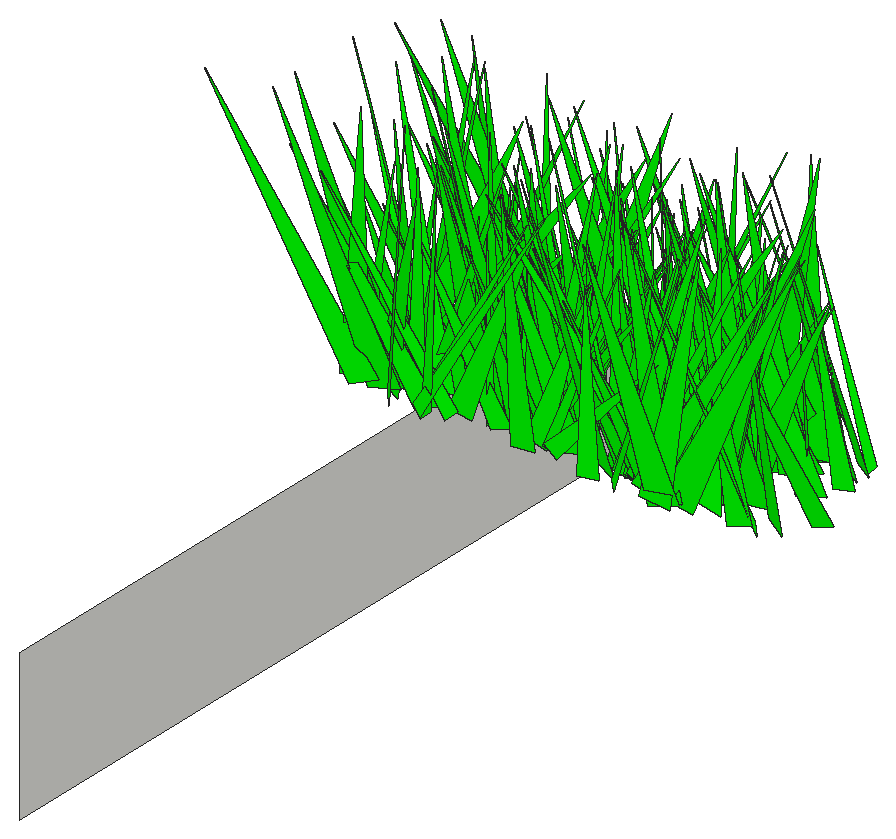
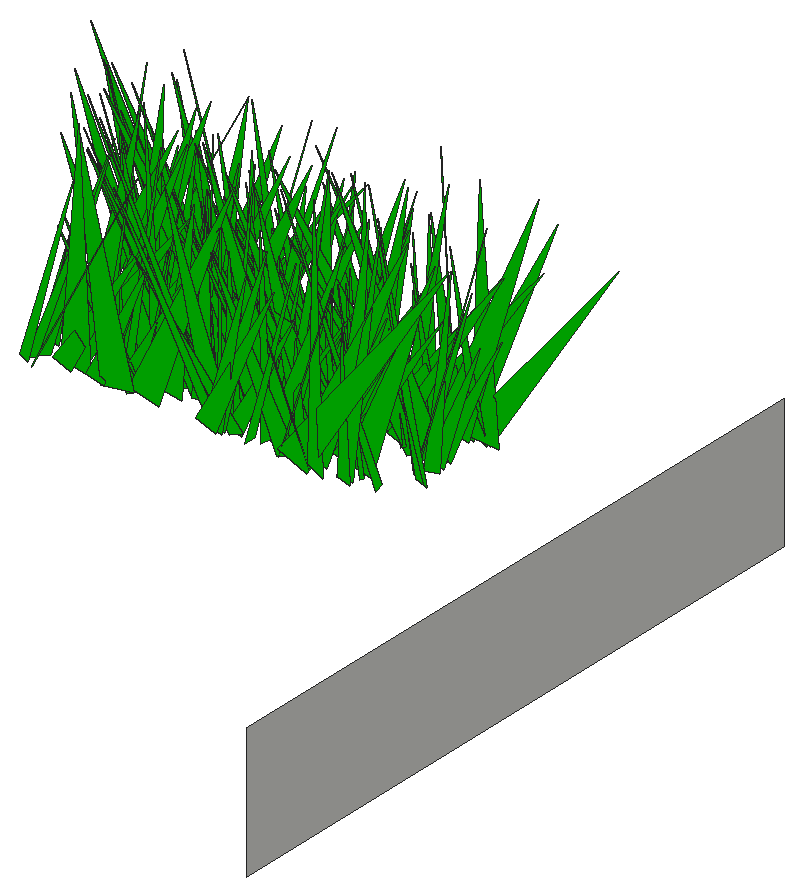
# SketchUp Ruby script. Lengths in inches.
U = 1.inch
M = Sketchup.active_model
def pt(a) = Geom::Point3d.new(a.map { |v| v * U })
def face(e, loops, mat)
  f = e.add_face(loops[0].map { |a| pt(a) })
  loops[1..].each { |l| e.add_face(l.map { |a| pt(a) }).erase! }
  f.material = f.back_material = mat if mat
  f
end
# faces: each face lists its corners as indices into pts; further lists are holes
def faces(e, pts, list, mat = nil) = list.each { |f| face(e, (f[0].is_a?(Array) ? f : [f]).map { |l| l.map { |i| pts[i] } }, mat) }
# xy, xz, yz: faces in a plane at the given z, y or x. An outline is a flat list of corners, or four numbers for a rectangle; further outlines are holes
def ring(l) = l.size == 4 ? [[l[0], l[1]], [l[2], l[1]], [l[2], l[3]], [l[0], l[3]]] : l.each_slice(2).to_a
def flat(e, list, mat, &to3) = list.each { |f| face(e, (f[0].is_a?(Array) ? f : [f]).map { |l| ring(l).map { |u, v| to3.(u, v) } }, mat) }
def xy(e, z, list, mat = nil) = flat(e, list, mat) { |x, y| [x, y, z] }
def xz(e, y, list, mat = nil) = flat(e, list, mat) { |x, z| [x, y, z] }
def yz(e, x, list, mat = nil) = flat(e, list, mat) { |y, z| [x, y, z] }
def lines(e, pts, list) = list.each { |a, b| e.add_line(pt(pts[a]), pt(pts[b])) }
# prism: a flat outline (further loops are holes) pulled along v
def prism(e, loops, v, mat = nil)
  f = face(e, loops, mat); d = Geom::Vector3d.new(v.map { |x| x * U })
  f.pushpull(f.normal.samedirection?(d) ? d.length : -d.length)
end
def box(e, o, s, mat = nil) = prism(e, [[o, [o[0] + s[0], o[1], o[2]], [o[0] + s[0], o[1] + s[1], o[2]], [o[0], o[1] + s[1], o[2]]]], [0, 0, s[2]], mat)
def at(x, y, z, deg = 0) = Geom::Transformation.translation(pt([x, y, z])) * Geom::Transformation.rotation(ORIGIN, Z_AXIS, deg.degrees)
def axes(o, x, y, z) = Geom::Transformation.new([*x, 0, *y, 0, *z, 0, *pt(o).to_a, 1])
def part(name) = M.definitions.add(name)
# library, detail: a bought-in or finely detailed component or shape, given as its bounding box
def library(name, o, s) = part(name).tap { |d| box(d.entities, o, s) }
def detail(e, o, s) = box(e.add_group.entities, o, s)
def put(e, d, t, mat = nil) = e.add_instance(d, t).tap { |i| i.material = mat if mat }
def group(e, t, mat = nil) = e.add_group.tap { |g| g.transformation = t; g.material = mat if mat }.entities
root = M.entities
M.materials.add("[0065_Lime]").color = [0, 255, 0]
c1 = part("fur_instance\#9")
p = [[0.8125,0,1.79],[0.67,-0.02,1.48],[0,-0.11,0],[0,0.11,0]]
faces(c1.entities,p,[[0,1,2,3]])
yz(root,5.71,[[0,-11.8125,39.75,-3.9375]])
put(root,c1,axes([8.52,19.14,1.48],[-4.51597,1.0152,0.75582],[-6.76232,-0.52719,-3.00512],[-2.70756,-0.37656,6.24484]),"[0065_Lime]")
put(root,c1,axes([9.53,19.26,1.48],[-0.92745,-1.18344,1.15572],[8.13091,-0.06085,2.2291],[-2.61483,0.23052,6.52155]),"[0065_Lime]")
put(root,c1,axes([8.54,21.75,1.48],[0.14236,-0.67611,0.80396],[4.52504,0.07211,1.50186],[-1.91106,0.12037,3.61603]),"[0065_Lime]")
put(root,c1,axes([8.66,23.4,1.48],[-8.88567,-0.25424,1.35395],[1.25522,-1.22333,-2.24699],[2.11392,-0.34227,7.02545]),"[0065_Lime]")
put(root,c1,axes([8.39,22.4,1.48],[-0.17151,-0.64742,0.31901],[4.46442,-0.00882,0.98829],[-1.20447,0.0595,3.61774]),"[0065_Lime]")
put(root,c1,axes([9.04,22.44,1.48],[-6.57212,0.41088,0.28365],[-2.7373,-0.89658,1.55629],[1.0858,0.22672,5.64032]),"[0065_Lime]")
put(root,c1,axes([9.7,19.55,1.48],[-0.1146,-1.28054,1.0583],[8.86048,0.03424,2.02291],[-2.49622,0.18031,7.13186]),"[0065_Lime]")
put(root,c1,axes([8.04,23.1,1.48],[-4.80678,-0.70041,0.91441],[4.7596,-0.69264,-1.22373],[1.85882,-0.03767,5.49804]),"[0065_Lime]")
put(root,c1,axes([11.95,19.03,1.48],[-4.72071,0.76903,0.39332],[-5.14246,-0.58693,-2.38257],[-1.93422,-0.31647,5.37455]),"[0065_Lime]")
put(root,c1,axes([7.86,19.42,1.48],[5.30316,-0.969,1.02],[6.74982,0.76558,1.15187],[-1.88838,0.01526,6.98171]),"[0065_Lime]")
put(root,c1,axes([10.86,25.02,1.48],[-2.71894,-1.0235,1.49211],[7.41679,-0.32251,1.5292],[-1.18715,0.32924,6.13636]),"[0065_Lime]")
put(root,c1,axes([8.25,19.28,1.48],[5.38611,0.66899,0.37338],[-4.41146,0.73237,-1.86579],[-1.84817,0.2015,5.54166]),"[0065_Lime]")
put(root,c1,axes([12.25,21.2,1.48],[-0.93493,-0.96245,1.99029],[6.42475,0.0532,2.8589],[-3.40916,0.3642,4.84194]),"[0065_Lime]")
put(root,c1,axes([7.98,24.05,1.48],[7.33829,0.65143,1.33023],[-4.37612,1.05375,-1.31921],[-2.23967,0.07548,6.9361]),"[0065_Lime]")
put(root,c1,axes([12.09,24.75,1.48],[-4.89413,0.62544,0.37384],[-4.32649,-0.637,-1.76465],[-1.14195,-0.26712,5.0835]),"[0065_Lime]")
put(root,c1,axes([13.77,26.3,1.48],[-3.51472,-1.22749,0.2766],[8.07714,-0.43627,3.03249],[-3.34436,0.23638,7.03326]),"[0065_Lime]")
put(root,c1,axes([11.29,21.7,1.48],[-1.10307,-0.63213,1.01067],[4.39567,-0.08044,1.48842],[-1.56819,0.21918,3.46114]),"[0065_Lime]")
put(root,c1,axes([7.87,24.19,1.48],[9.02923,-0.23707,1.46941],[1.26598,1.26925,1.71479],[-2.12296,-0.25139,7.27216]),"[0065_Lime]")
put(root,c1,axes([10.75,26.15,1.48],[-6.90175,-0.73018,1.53288],[5.0802,-1.00487,-0.90557],[2.17833,0.03003,6.96867]),"[0065_Lime]")
put(root,c1,axes([13.17,19.14,1.48],[-6.55039,0.35414,0.43805],[-2.49164,-0.81745,-2.50688],[-0.65837,-0.42978,5.12908]),"[0065_Lime]")
put(root,c1,axes([9.55,20.76,1.48],[5.24517,0.61285,0.37116],[-3.95773,0.70463,-1.98125],[-1.8885,0.22546,5.18298]),"[0065_Lime]")
put(root,c1,axes([11.61,20.6,1.48],[-8.02681,0.63334,1.21574],[-4.33342,-1.14566,1.0688],[1.94162,0.06133,7.41134]),"[0065_Lime]")
put(root,c1,axes([12,23.47,1.48],[0.00491,-0.81088,1.79265],[5.85718,0.09899,1.48978],[-1.96232,0.29344,4.45122]),"[0065_Lime]")
put(root,c1,axes([13.33,25.51,1.48],[-2.13529,1.23511,1.47302],[-8.6321,-0.21112,-2.34727],[-2.45463,-0.33197,6.97314]),"[0065_Lime]")
put(root,c1,axes([13.64,24.76,1.48],[-2.97825,-0.76492,0.9224],[5.21144,-0.32095,2.21457],[-1.93893,0.31228,4.53548]),"[0065_Lime]")
put(root,c1,axes([9.54,19.4,1.48],[-4.12303,-0.93043,0.23604],[5.76195,-0.52692,-3.00694],[3.2753,-0.24428,5.58699]),"[0065_Lime]")
put(root,c1,axes([10.28,20.8125,1.48],[-1.74906,-0.67558,0.04949],[4.57049,-0.23643,-1.27519],[1.49314,-0.06767,3.96131]),"[0065_Lime]")
put(root,c1,axes([10.2,18.69,1.48],[-7.80887,-0.33604,3.12821],[1.23428,-1.19432,-2.26054],[4.35726,-0.26392,6.24658]),"[0065_Lime]")
put(root,c1,axes([10.73,19.87,1.48],[-5.16109,0.39853,3.17519],[-4.06968,-0.79103,-1.04984],[2.59212,-0.44843,4.67376]),"[0065_Lime]")
put(root,c1,axes([10.71,26.29,1.48],[4.13664,-0.44364,0.53641],[2.83698,0.57217,1.38184],[-1.53443,-0.13814,4.00095]),"[0065_Lime]")
put(root,c1,axes([10.16,25.64,1.48],[5.76638,0.14354,1.65664],[-1.58452,0.81226,1.29083],[-1.6373,-0.28053,4.58525]),"[0065_Lime]")
put(root,c1,axes([12.85,22.17,1.48],[2.25168,1.20305,2.13517],[-8.5324,0.40368,-1.66827],[-2.71834,-0.27056,7.00502]),"[0065_Lime]")
put(root,c1,axes([10.55,22.08,1.48],[3.82403,0.16991,1.08744],[-1.59634,0.52385,0.97141],[-0.83732,-0.22273,3.11433]),"[0065_Lime]")
put(root,c1,axes([12.38,24.16,1.48],[3.26238,1.02924,2.0799],[-7.34786,0.535,-1.24568],[-2.48954,-0.23028,6.40217]),"[0065_Lime]")
put(root,c1,axes([8.72,22.16,1.48],[2.49265,1.12942,1.40234],[-7.98484,0.27249,2.03678],[1.95376,-0.32729,6.535]),"[0065_Lime]")
put(root,c1,axes([11.73,22.16,1.48],[-5.38252,-0.24176,1.5364],[0.68863,-0.73331,-2.27042],[2.46041,-0.32365,3.99656]),"[0065_Lime]")
put(root,c1,axes([11.08,24.76,1.48],[5.87705,-0.3291,0.76024],[1.70229,0.76351,2.36835],[-1.86039,-0.34103,4.56871]),"[0065_Lime]")
put(root,c1,axes([12.29,18.54,1.48],[5.85026,0.55929,0.97233],[-3.04973,0.77481,-2.7932],[-2.8231,0.32199,5.03236]),"[0065_Lime]")
put(root,c1,axes([12.02,21.33,1.48],[3.45962,0.59945,0.27658],[-4.04081,0.4778,-1.25847],[-1.40947,0.10159,4.28681]),"[0065_Lime]")
put(root,c1,axes([9.04,25.82,1.48],[9.00581,0.29151,1.30551],[-2.57623,1.13462,3.2688],[-0.49281,-0.6041,6.7694]),"[0065_Lime]")
put(root,c1,axes([13.5625,23.2,1.48],[0.41564,-0.69447,0.03329],[4.68844,0.05723,1.27394],[-1.56396,-0.01301,3.82785]),"[0065_Lime]")
put(root,c1,axes([14.9,20.67,1.48],[-9.0282,-0.11103,1.59013],[1.50199,-1.18634,2.8667],[1.47982,0.52675,6.79149]),"[0065_Lime]")
put(root,c1,axes([13.49,20.99,1.48],[2.41747,-1.08088,0.01398],[7.39832,0.32741,1.79122],[-2.10575,-0.09056,6.30927]),"[0065_Lime]")
put(root,c1,axes([9.15,21.7,1.48],[2.60344,0.683,0.40678],[-4.0014,0.25231,2.74862],[2.80439,-0.27406,3.5442]),"[0065_Lime]")
put(root,c1,axes([12.3,26.41,1.48],[8.37035,-0.55491,1.57527],[2.96399,1.14389,3.08182],[-3.24961,-0.38598,6.86854]),"[0065_Lime]")
put(root,c1,axes([14.71,25.96,1.48],[-6.89277,0.09509,0.79888],[-0.3282,-0.92938,1.83337],[1.14666,0.3056,5.32696]),"[0065_Lime]")
put(root,c1,axes([13.4,23.63,1.48],[-4.04851,-0.00151,1.22127],[0.64281,-0.55006,1.38709],[1.3569,0.25608,2.98674]),"[0065_Lime]")
put(root,c1,axes([15.44,19.57,1.48],[-2.28354,0.71758,0.28524],[-4.82771,-0.28399,-1.63183],[-1.70136,-0.15729,4.24757]),"[0065_Lime]")
put(root,c1,axes([10.88,20.86,1.48],[7.55042,-0.47397,0.27797],[3.24255,1.04379,1.36389],[-0.99004,-0.19613,6.58688]),"[0065_Lime]")
put(root,c1,axes([16.12,20.47,1.48],[-3.81413,-0.77301,1.85642],[5.88572,-0.43097,1.98756],[-0.91089,0.45206,5.06931]),"[0065_Lime]")
put(root,c1,axes([13.43,22.12,1.48],[4.49135,-0.41416,0.66232],[2.59175,0.6235,1.436],[-1.62259,-0.15048,4.12702]),"[0065_Lime]")
put(root,c1,axes([13.64,23.21,1.48],[-4.1807,0.3084,1.23402],[-1.6634,-0.61111,1.389],[2.086,0.13077,3.58078]),"[0065_Lime]")
put(root,c1,axes([10.24,21.75,1.48],[4.09063,0.70798,0.20575],[-4.5194,0.49397,2.49387],[2.2415,-0.29608,4.65274]),"[0065_Lime]")
put(root,c1,axes([9.5625,22.0625,1.48],[2.5963,1.09286,2.35775],[-7.43893,0.11711,3.60096],[3.68129,-0.53412,5.61375]),"[0065_Lime]")
put(root,c1,axes([12.93,26.23,1.48],[4.17456,0.20644,0.24318],[-1.28002,0.55547,-1.26266],[-0.78058,0.19317,3.37107]),"[0065_Lime]")
put(root,c1,axes([14.375,20.41,1.48],[6.01675,0.77907,1.63573],[-4.94463,0.88638,-2.1125],[-3.21463,0.09478,6.31094]),"[0065_Lime]")
put(root,c1,axes([13.99,23.44,1.48],[4.68309,0.12287,2.12125],[-1.719,0.6956,1.16081],[-2.1472,-0.2889,3.69717]),"[0065_Lime]")
put(root,c1,axes([15.82,24.58,1.48],[-2.8334,-0.89119,1.44388],[6.54685,-0.3516,1.22824],[-0.71622,0.31162,5.51512]),"[0065_Lime]")
put(root,c1,axes([16.13,20.16,1.48],[-4.02935,-0.9593,2.013],[7.24625,-0.50535,1.52712],[-0.47165,0.43143,6.26472]),"[0065_Lime]")
put(root,c1,axes([16.54,24.29,1.48],[-5.49409,0.14275,0.08975],[-1.00323,-0.7374,-1.3325],[-0.19417,-0.22909,4.34498]),"[0065_Lime]")
put(root,c1,axes([11.63,18.93,1.48],[6.96665,0.31379,0.36258],[-2.27528,0.95111,1.3437],[0.09165,-0.24008,5.79707]),"[0065_Lime]")
put(root,c1,axes([14.69,19.83,1.48],[5.57745,-0.27415,1.43426],[1.19173,0.78139,1.93868],[-2.34423,-0.25504,4.39799]),"[0065_Lime]")
put(root,c1,axes([16.5,26.02,1.48],[-7.04698,0.30872,0.64956],[-1.89783,-0.96364,1.72416],[1.36483,0.25402,5.75134]),"[0065_Lime]")
put(root,c1,axes([14.49,24.81,1.48],[-2.29166,-0.51115,0.22563],[3.31371,-0.3109,-1.3328],[1.52593,-0.09249,3.23316]),"[0065_Lime]")
put(root,c1,axes([17.05,20.16,1.48],[-3.17395,-0.57364,0.51178],[4.07145,-0.4157,1.09338],[-0.6961,0.18419,4.06157]),"[0065_Lime]")
put(root,c1,axes([11.74,18.625,1.48],[7.66634,0.35493,0.19048],[-2.50408,1.04211,1.61392],[0.40557,-0.2749,6.3642]),"[0065_Lime]")
put(root,c1,axes([13.32,19.49,1.48],[4.55521,-0.7039,0.8959],[5.12184,0.61336,-1.08206],[0.27057,0.23968,5.40009]),"[0065_Lime]")
put(root,c1,axes([16.33,23.36,1.48],[7.70292,-0.44018,2.74672],[1.5377,1.11728,3.14665],[-4.3418,-0.38524,5.98747]),"[0065_Lime]")
put(root,c1,axes([12.02,23.78,1.48],[5.7024,0.51738,0.07898],[-3.36031,0.72049,2.37175],[1.50814,-0.35092,4.98591]),"[0065_Lime]")
put(root,c1,axes([15.87,25.56,1.48],[6.42184,-0.14988,2.81865],[2.12568,0.95797,-1.49745],[-2.93715,0.36562,5.07901]),"[0065_Lime]")
put(root,c1,axes([14.69,23.95,1.48],[-0.98557,1.08875,0.87105],[-7.6069,-0.16872,1.372],[1.82083,-0.11556,6.2033]),"[0065_Lime]")
put(root,c1,axes([16.68,24.31,1.48],[-5.48029,-0.51583,0.37851],[3.28972,-0.73269,-1.9446],[1.6941,-0.24588,5.0006]),"[0065_Lime]")
put(root,c1,axes([17.65,25.78,1.48],[-1.66406,-0.64022,0.09718],[4.42274,-0.22251,0.98748],[-1.10098,0.07381,3.81991]),"[0065_Lime]")
put(root,c1,axes([16,21.53,1.48],[3.40175,-1.04621,0.40794],[7.31725,0.48285,1.12339],[-1.46396,-0.01762,6.5629]),"[0065_Lime]")
put(root,c1,axes([12.69,24.53,1.48],[4.62258,-1.01151,0.2415],[7.00165,0.61904,-1.79019],[1.69797,0.20113,6.72445]),"[0065_Lime]")
put(root,c1,axes([13.9,21.72,1.48],[3.47793,-0.48907,0.50837],[3.40501,0.42994,-1.55281],[0.95405,0.24839,3.68875]),"[0065_Lime]")
put(root,c1,axes([17.74,20.77,1.48],[-6.59474,-0.29254,0.84748],[1.81984,-0.92208,-1.29581],[1.45182,-0.17299,5.47391]),"[0065_Lime]")
put(root,c1,axes([17.17,18.83,1.48],[3.20094,0.84632,2.02875],[-6.13144,0.52346,-0.91648],[-2.21378,-0.22611,5.47176]),"[0065_Lime]")
put(root,c1,axes([14.18,26.12,1.48],[3.04422,-0.76222,0.33004],[5.28546,0.39905,-1.37437],[1.28548,0.16429,4.86937]),"[0065_Lime]")
put(root,c1,axes([19.07,19.81,1.48],[-2.15391,0.85559,1.06284],[-6.02122,-0.23654,-1.69296],[-1.58939,-0.26337,4.97324]),"[0065_Lime]")
put(root,c1,axes([18.95,26.2,1.48],[-0.24233,0.79074,1.33555],[-5.42007,0.05773,-1.79607],[-2.23285,-0.22596,4.21486]),"[0065_Lime]")
put(root,c1,axes([18.57,20.2,1.48],[2.6144,0.97004,2.07295],[-6.70575,0.47056,-1.78289],[-3.03038,-0.20439,5.73364]),"[0065_Lime]")
put(root,c1,axes([14.93,23.24,1.48],[0.60212,0.75738,0.49855],[-5.05075,0.04666,1.6609],[1.97915,-0.11135,4.08692]),"[0065_Lime]")
put(root,c1,axes([18.52,26.09,1.48],[-4.33642,0.6658,1.51044],[-5.0832,-0.58317,-1.04194],[0.24485,-0.31512,5.11962]),"[0065_Lime]")
put(root,c1,axes([18.59,26.18,1.48],[0.96901,0.76025,1.42682],[-5.43354,0.19764,-1.0872],[-1.68099,-0.20058,4.3367]),"[0065_Lime]")
put(root,c1,axes([16.92,23.49,1.48],[5.89619,0.791,0.90812],[-5.37717,0.84006,-1.41937],[-2.005,0.07319,6.47712]),"[0065_Lime]")
put(root,c1,axes([15.11,25.13,1.48],[5.44388,-0.9912,1.83413],[7.39986,0.71269,-1.62604],[0.28992,0.42147,7.063]),"[0065_Lime]")
put(root,c1,axes([18.28,22.1,1.48],[1.21948,-1.0478,0.48649],[7.36376,0.18314,1.00402],[-1.3172,0.05374,6.06339]),"[0065_Lime]")
put(root,c1,axes([13.87,24.05,1.48],[8.12448,0.55349,0.5173],[-3.95019,1.08727,2.06616],[0.56173,-0.35938,7.04766]),"[0065_Lime]")
put(root,c1,axes([18.51,22.11,1.48],[4.9532,0.68925,0.32577],[-3.78832,0.58496,-3.36104],[-3.14147,0.38135,4.56675]),"[0065_Lime]")
put(root,c1,axes([21.12,20.95,1.48],[-7.61214,0.41528,0.77912],[-3.10394,-1.00153,-2.17679],[-0.1316,-0.39898,6.27527]),"[0065_Lime]")
put(root,c1,axes([16.91,20.72,1.48],[6.07858,0.79409,0.71559],[-5.49002,0.86072,-1.15017],[-1.60306,0.06339,6.6524]),"[0065_Lime]")
put(root,c1,axes([18.42,25.09,1.48],[8.11333,-0.28978,2.87345],[0.54432,1.16931,2.93449],[-4.05407,-0.42292,6.14458]),"[0065_Lime]")
put(root,c1,axes([21.22,22.83,1.48],[-0.0959,1.26545,2.06522],[-8.71312,0.11796,-2.6897],[-3.41024,-0.33697,6.81409]),"[0065_Lime]")
put(root,c1,axes([18.42,24.93,1.48],[-4.0699,0.59218,1.00747],[-4.03607,-0.59779,0.98637],[1.73333,-0.00149,4.66234]),"[0065_Lime]")
put(root,c1,axes([17.75,20.57,1.48],[-2.38096,0.7267,0.44801],[-4.87591,-0.34152,1.41733],[1.80943,0.03594,4.40882]),"[0065_Lime]")
put(root,c1,axes([15.7,24.66,1.48],[5.71354,0.41429,0.15378],[-2.91512,0.78116,1.14195],[0.48012,-0.18727,5.10356]),"[0065_Lime]")
put(root,c1,axes([17.34,19.51,1.48],[0.09973,0.74013,1.16518],[-5.26071,-0.04067,1.16348],[1.45594,-0.19763,4.12416]),"[0065_Lime]")
put(root,c1,axes([16.4,23.3,1.48],[3.50553,0.60675,0.37787],[-4.21361,0.45487,1.38897],[1.05165,-0.19999,4.30553]),"[0065_Lime]")
put(root,c1,axes([17.16,20.46,1.48],[2.50517,-0.48253,0.39816],[3.38299,0.32114,-1.04162],[0.76627,0.15974,3.2969]),"[0065_Lime]")
put(root,c1,axes([20.96,19.52,1.48],[-7.43308,-0.74265,0.09237],[5.10424,-1.01544,-1.80452],[1.37541,-0.24511,7.19589]),"[0065_Lime]")
put(root,c1,axes([17.08,21.82,1.48],[4.51394,-0.4487,0.47947],[3.2111,0.59576,-1.31974],[0.48227,0.23291,4.29952]),"[0065_Lime]")
put(root,c1,axes([23.86,19.72,1.48],[-7.55702,0.55256,0.45368],[-3.66216,-0.90423,-3.45697],[-1.53717,-0.56225,6.00549]),"[0065_Lime]")
put(root,c1,axes([19.38,22.55,1.48],[5.89257,-0.70031,1.82599],[4.81059,0.88466,1.09782],[-2.59528,0.04976,6.18081]),"[0065_Lime]")
put(root,c1,axes([22.67,22.89,1.48],[-6.39879,0.95966,0.60157],[-6.83825,-0.87635,-1.28002],[-0.65348,-0.22642,7.50414]),"[0065_Lime]")
put(root,c1,axes([21.78,19.8125,1.48],[-9.09715,0.09459,1.29901],[-0.39391,-1.28059,1.29956],[1.68771,0.21099,7.30528]),"[0065_Lime]")
put(root,c1,axes([22.33,19.67,1.48],[-4.416,-0.64604,0.07079],[4.48389,-0.6012,1.21621],[-1.01984,0.15413,5.04075]),"[0065_Lime]")
put(root,c1,axes([17.12,21.49,1.48],[6.70773,0.00986,0.12097],[-0.02769,0.90829,-1.46372],[-0.16207,0.2527,5.25646]),"[0065_Lime]")
put(root,c1,axes([22.09,19.85,1.48],[-1.79777,-0.88309,0.27518],[6.01526,-0.22655,1.63889],[-1.85121,0.12145,5.05811]),"[0065_Lime]")
put(root,c1,axes([19.6,24.38,1.48],[6.36613,-0.10869,2.08487],[0.06988,0.93549,1.49298],[-2.67637,-0.2341,4.99816]),"[0065_Lime]")
put(root,c1,axes([17.96,19.5,1.48],[6.05892,-0.23996,0.84944],[1.88291,0.84198,-0.91596],[-0.67926,0.19355,5.03783]),"[0065_Lime]")
put(root,c1,axes([16.89,20.13,1.48],[4.42451,-0.5492,0.03176],[3.68651,0.58361,-1.62949],[1.29876,0.21439,4.5171]),"[0065_Lime]")
put(root,c1,axes([18.36,20.66,1.48],[8.33689,-0.54395,0.94778],[3.45356,1.15337,2.08145],[-2.10132,-0.26251,7.18114]),"[0065_Lime]")
put(root,c1,axes([18.33,25.85,1.48],[3.38953,-0.89243,1.33201],[6.54542,0.44377,-1.05748],[0.41788,0.28788,5.75943]),"[0065_Lime]")
put(root,c1,axes([17.64,23.85,1.48],[5.96023,-0.46701,0.64256],[3.4115,0.80214,-1.40167],[0.17724,0.2652,5.37103]),"[0065_Lime]")
put(root,c1,axes([17.33,25.96,1.48],[3.64067,0.5823,0.06313],[-3.79484,0.46248,1.85477],[1.66655,-0.21896,4.0855]),"[0065_Lime]")
put(root,c1,axes([20.04,23.68,1.48],[5.99339,-0.03413,1.99993],[0.82635,0.882,-1.13409],[-2.32837,0.22517,4.74547]),"[0065_Lime]")
put(root,c1,axes([22.9,25.83,1.48],[-0.54012,-1.15286,1.54114],[8.03809,0.00887,2.08637],[-2.50824,0.2767,6.35427]),"[0065_Lime]")
put(root,c1,axes([20.8125,18.59,1.48],[1.89627,0.78277,0.02171],[-5.4228,0.26029,-1.08832],[-1.27498,0.05713,4.66117]),"[0065_Lime]")
put(root,c1,axes([21.95,23.6,1.48],[-3.47813,-0.29125,0.8576],[2.32393,-0.42575,1.39094],[-0.08361,0.28204,2.98527]),"[0065_Lime]")
put(root,c1,axes([20.75,22.02,1.48],[3.87743,-0.67179,0.07295],[4.36699,0.50412,1.98537],[-1.94774,-0.20708,4.59656]),"[0065_Lime]")
put(root,c1,axes([20.59,24.09,1.48],[-7.86521,-0.25931,2.69613],[1.33199,-1.19259,-1.27254],[3.55214,-0.12696,6.447]),"[0065_Lime]")
put(root,c1,axes([20.62,24.42,1.48],[-3.82011,-0.82764,1.01387],[5.73641,-0.56335,-1.1091],[1.8272,0.03826,5.60166]),"[0065_Lime]")
put(root,c1,axes([19.54,23.47,1.48],[-1.28465,0.79365,1.70019],[-5.72052,-0.2547,1.12418],[1.88287,-0.23233,4.57547]),"[0065_Lime]")
put(root,c1,axes([20.43,23.3125,1.48],[6.35862,0.1381,1.92875],[-0.06165,0.89809,-2.0202],[-2.56604,0.32062,4.82798]),"[0065_Lime]")
put(root,c1,axes([21.95,23.25,1.48],[-6.46346,0.5085,2.0855],[-4.14582,-0.91893,-0.99326],[1.57525,-0.33203,5.94298]),"[0065_Lime]")
put(root,c1,axes([18.22,19.34,1.48],[2.94829,0.52874,0.24565],[-3.29329,0.33395,2.06554],[1.84503,-0.24882,3.29435]),"[0065_Lime]")
put(root,c1,axes([23.33,19.47,1.48],[-2.43351,-0.64341,0.39846],[4.40831,-0.30298,1.41944],[-1.33131,0.17283,3.97179]),"[0065_Lime]")
put(root,c1,axes([20.65,22.72,1.48],[3.58257,0.38797,0.25367],[-2.56619,0.48941,-1.1031],[-1.06545,0.12578,3.50985]),"[0065_Lime]")
put(root,c1,axes([22.16,24.9,1.48],[0.91206,0.93865,1.39069],[-6.7545,0.17034,-0.9217],[-1.38625,-0.21243,5.40597]),"[0065_Lime]")
put(root,c1,axes([22.04,21.95,1.48],[3.39012,-0.70905,1.98643],[5.09657,0.55685,0.90545],[-2.33461,0.18602,4.86115]),"[0065_Lime]")
put(root,c1,axes([18.49,26.06,1.48],[7.4207,-0.1667,0.42383],[1.28389,1.0034,-1.64841],[-0.17476,0.293,5.88629]),"[0065_Lime]")
put(root,c1,axes([22.82,21.36,1.48],[-0.43333,0.62229,0.55221],[-4.27707,-0.02892,-1.1285],[-1.33393,-0.10941,3.439]),"[0065_Lime]")
put(root,c1,axes([24.35,25.38,1.48],[-6.00986,0.50917,0.2512],[-3.61271,-0.82628,-1.06508],[-0.41692,-0.17973,5.60807]),"[0065_Lime]")
put(root,c1,axes([23.3125,24.18,1.48],[-4.69701,0.48117,1.24468],[-3.73888,-0.62794,-1.20102],[0.29648,-0.29588,4.57304]),"[0065_Lime]")
put(root,c1,axes([23.28,25.59,1.48],[-6.15326,-0.23557,1.18735],[1.41549,-0.88072,-1.00176],[1.71398,-0.11838,5.08994]),"[0065_Lime]")
put(root,c1,axes([19.16,25.43,1.48],[9.29072,-0.12072,0.69166],[1.01707,1.28117,-1.54656],[-0.65315,0.27791,7.43018]),"[0065_Lime]")
put(root,c1,axes([21.09,20.05,1.48],[6.13723,-0.60435,0.13964],[4.12209,0.83731,1.56342],[-1.23922,-0.20785,5.89201]),"[0065_Lime]")
put(root,c1,axes([24.6875,18.72,1.48],[2.2656,-1.08197,0.72255],[7.13818,0.34194,2.3484],[-3.02056,-0.00348,6.0917]),"[0065_Lime]")
put(root,c1,axes([24.53,19.08,1.48],[2.13667,1.06298,2.53681],[-7.81954,0.39866,-1.23989],[-2.40977,-0.35109,6.27266]),"[0065_Lime]")
put(root,c1,axes([20.67,22.3,1.48],[2.02176,-1.09692,0.01344],[7.53735,0.27368,-1.7102],[2.03135,0.07624,6.33235]),"[0065_Lime]")
put(root,c1,axes([22.53,19.69,1.48],[-2.29915,0.87751,1.85902],[-6.29563,-0.39666,1.12239],[2.14158,-0.22399,5.29532]),"[0065_Lime]")
put(root,c1,axes([25.08,20.27,1.48],[1.56928,-0.65387,2.05959],[4.69607,0.34344,1.28619],[-2.4518,0.2393,3.78176]),"[0065_Lime]")
put(root,c1,axes([23.125,24.45,1.48],[7.35719,0.52698,3.02332],[-4.52237,1.09126,0.90767],[-2.72532,-0.38821,6.65546]),"[0065_Lime]")
put(root,c1,axes([20.95,24.11,1.48],[3.61961,0.82989,0.62093],[-5.7258,0.45051,1.90769],[1.63639,-0.2593,5.30162]),"[0065_Lime]")
put(root,c1,axes([24.57,25.07,1.48],[-7.36013,-0.54153,1.22766],[3.22407,-1.02148,-2.30968],[2.59526,-0.26681,6.35092]),"[0065_Lime]")
put(root,c1,axes([21.89,19.6875,1.48],[7.11167,-0.62344,1.95251],[4.95551,0.97243,-1.53783],[-0.94315,0.40839,6.64246]),"[0065_Lime]")
put(root,c1,axes([26.37,21.83,1.48],[-3.48756,0.55443,0.51334],[-3.85091,-0.43496,-1.5685],[-1.06621,-0.24256,3.98595]),"[0065_Lime]")
put(root,c1,axes([25.67,26.02,1.48],[-1.01541,-0.70529,0.3188],[4.87151,-0.12347,1.11339],[-1.27064,0.09027,4.01385]),"[0065_Lime]")
put(root,c1,axes([20.82,23.89,1.48],[1.48701,1.00085,1.61784],[-6.6873,0.06029,2.81708],[3.15709,-0.34371,5.20509]),"[0065_Lime]")
put(root,c1,axes([22,18.73,1.48],[8.80297,0.1664,1.42498],[-1.5176,1.2311,1.38578],[-1.47247,-0.27404,7.0908]),"[0065_Lime]")
put(root,c1,axes([26.91,24.02,1.48],[1.25141,1.06442,3.09469],[-7.74316,0.36345,-2.11725],[-3.44952,-0.42969,5.87529]),"[0065_Lime]")
put(root,c1,axes([20.43,21.65,1.48],[3.15387,1.19364,0.71562],[-8.01819,0.36852,2.7835],[2.93958,-0.27547,6.82469]),"[0065_Lime]")
put(root,c1,axes([27.87,24.53,1.48],[-1.01053,-0.86953,2.06902],[5.86402,0.05892,2.72469],[-3.22104,0.38006,4.31128]),"[0065_Lime]")
put(root,c1,axes([25.7,20.4,1.48],[-6.03092,0.62583,0.43279],[-4.22135,-0.83428,1.50453],[1.51633,0.16656,5.90981]),"[0065_Lime]")
put(root,c1,axes([21.97,23.74,1.48],[4.55289,-0.68883,0.67773],[4.89116,0.59183,-1.5838],[0.89525,0.2697,5.20637]),"[0065_Lime]")
put(root,c1,axes([24.99,22.25,1.48],[3.97316,-0.14517,1.44961],[0.20577,0.56931,1.53734],[-2.04964,-0.22426,2.96437]),"[0065_Lime]")
put(root,c1,axes([22.375,22.48,1.48],[2.16696,0.77902,0.29908],[-5.26637,0.27031,1.65314],[1.77069,-0.14939,4.55076]),"[0065_Lime]")
put(root,c1,axes([23.09,19.33,1.48],[2.99533,0.54109,0.38067],[-3.82062,0.39717,0.97347],[0.67041,-0.15405,3.84697]),"[0065_Lime]")
put(root,c1,axes([21.89,23.99,1.48],[2.84893,-0.95187,0.41384],[6.45105,0.35481,-2.03694],[2.12845,0.1987,5.61979]),"[0065_Lime]")
put(root,c1,axes([26.01,20.18,1.48],[-4.84006,-0.12597,0.61921],[0.57982,-0.64973,-1.43061],[1.02323,-0.2277,3.73963]),"[0065_Lime]")
put(root,c1,axes([24.41,23.3,1.48],[-3.13663,1.01918,0.59999],[-6.9909,-0.45248,1.57452],[2.06826,0.0162,6.23192]),"[0065_Lime]")
put(root,c1,axes([24.76,25.04,1.48],[3.92169,-0.19014,0.91451],[0.9973,0.55825,1.05964],[-1.44928,-0.13036,3.20381]),"[0065_Lime]")
put(root,c1,axes([25.58,25.69,1.48],[-5.81468,-0.50731,0.58114],[2.94549,-0.75404,-2.55722],[2.20647,-0.33031,4.94519]),"[0065_Lime]")
put(root,c1,axes([22.34,19.68,1.48],[8.26557,-0.26119,1.08203],[2.22148,1.08308,-2.46705],[-0.53821,0.45919,6.4345]),"[0065_Lime]")
put(root,c1,axes([27.77,25.84,1.48],[-0.46133,-0.72727,1.58436],[4.94512,0.06868,2.00912],[-2.47525,0.27276,3.71857]),"[0065_Lime]")
put(root,c1,axes([22.09,23.46,1.48],[7.69522,0.14462,0.06252],[-1.01823,1.05056,1.48858],[0.16857,-0.25629,6.13718]),"[0065_Lime]")
put(root,c1,axes([24.26,18.66,1.48],[-2.22643,0.95176,2.66961],[-7.16146,-0.41584,1.01612],[2.31546,-0.37099,5.70972]),"[0065_Lime]")
put(root,c1,axes([27.33,21.1,1.48],[-1.68254,1.08291,2.27179],[-8.08741,-0.15399,-1.50329],[-1.33628,-0.43151,6.23771]),"[0065_Lime]")
put(root,c1,axes([27.72,21.05,1.48],[-2.35031,-1.17769,0.94657],[8.33561,-0.29309,1.47479],[-1.45396,0.2234,6.92495]),"[0065_Lime]")
put(root,c1,axes([28.89,19.57,1.48],[-9.12395,-0.2365,0.02394],[1.60508,-1.22919,-2.14949],[0.50711,-0.36445,7.23417]),"[0065_Lime]")
put(root,c1,axes([23.51,25.83,1.48],[3.39015,-0.52227,0.80215],[3.73014,0.40176,-1.66528],[0.93432,0.29107,3.73783]),"[0065_Lime]")
put(root,c1,axes([23.73,25.51,1.48],[3.83185,-0.5126,0.57547],[3.65993,0.49594,-1.3215],[0.64253,0.23205,4.09552]),"[0065_Lime]")
put(root,c1,axes([26.82,21.27,1.48],[1.28182,1.24388,1.52884],[-8.89935,0.22165,-1.1061],[-1.64141,-0.23036,7.19095]),"[0065_Lime]")
put(root,c1,axes([28.78,26.75,1.48],[-8.04702,-0.16843,0.12981],[1.13919,-1.10655,-1.38658],[0.40553,-0.23373,6.47088]),"[0065_Lime]")
put(root,c1,axes([24.34,26.04,1.48],[-0.75126,-1.25547,1.97192],[9.01922,-0.17632,-1.48822],[2.08748,0.30999,7.1397]),"[0065_Lime]")
put(root,c1,axes([28.99,23.13,1.48],[-5.52222,0.94574,0.82614],[-6.74609,-0.73602,-1.60206],[-0.90543,-0.28421,6.8979]),"[0065_Lime]")
put(root,c1,axes([27.47,24.03,1.48],[2.28729,-1.08923,2.54526],[7.97454,0.42103,1.29611],[-2.50702,0.34549,6.44497]),"[0065_Lime]")
put(root,c1,axes([26.1875,19.7,1.48],[-4.60638,0.96084,0.27918],[-6.53461,-0.63436,1.82083],[2.0427,0.1374,6.45441]),"[0065_Lime]")
put(root,c1,axes([25.91,20.41,1.48],[4.41809,0.04852,1.25468],[0.35807,0.59598,-1.60651],[-1.53956,0.27785,3.22691]),"[0065_Lime]")
put(root,c1,axes([26.15,22.3,1.48],[-5.8736,0.59455,1.7377],[-3.70322,-0.87398,1.73827],[2.95847,0.0864,5.62579]),"[0065_Lime]")
put(root,c1,axes([24.22,19.98,1.48],[2.40097,0.92452,1.09803],[-6.56392,0.2803,1.58801],[1.42332,-0.2669,5.47119]),"[0065_Lime]")
put(root,c1,axes([27.07,25.6875,1.48],[2.82479,1.21946,0.70353],[-8.53678,0.41276,-1.29535],[-1.78467,-0.04422,7.30973]),"[0065_Lime]")
put(root,c1,axes([23.96,23.04,1.48],[1.27507,-1.19249,2.42395],[8.66017,0.04854,-2.21387],[2.42925,0.45287,6.62008]),"[0065_Lime]")
put(root,c1,axes([24,21.57,1.48],[8.10325,-0.01879,0.59197],[0.27081,1.12184,-1.25976],[-0.6886,0.22013,6.4707]),"[0065_Lime]")
put(root,c1,axes([23.3,19.21,1.48],[6.35711,-0.76145,0.92763],[5.46373,0.82275,-2.14326],[0.90157,0.38303,6.44779]),"[0065_Lime]")
put(root,c1,axes([28.22,19.33,1.48],[2.00572,0.92121,0.58095],[-6.1329,0.29912,-1.88462],[-2.4242,0.00544,5.24849]),"[0065_Lime]")
put(root,c1,axes([25.29,20.88,1.48],[8.51797,0.1396,1.3921],[-0.15274,1.10594,-3.09789],[-1.97298,0.51708,6.24996]),"[0065_Lime]")
put(root,c1,axes([29.26,26.21,1.48],[-7.90354,-0.51873,0.39289],[3.5311,-1.09491,-1.44215],[1.17994,-0.19795,6.94743]),"[0065_Lime]")
put(root,c1,axes([25.1,21.06,1.48],[8.31287,0.15155,1.40125],[-1.40339,1.16525,1.28561],[-1.47012,-0.25543,6.69617]),"[0065_Lime]")
put(root,c1,axes([28.95,25.6875,1.48],[-7.51125,-0.64548,0.05204],[4.31543,-0.99726,-2.37607],[1.57556,-0.34576,6.75609]),"[0065_Lime]")
put(root,c1,axes([30.93,21.4375,1.48],[-3.47105,-0.85468,0.17134],[5.71962,-0.44646,2.03826],[-2.07986,0.19861,5.31929]),"[0065_Lime]")
put(root,c1,axes([26.48,20.35,1.48],[6.56478,0.64135,1.86862],[-4.97498,0.92214,0.95868],[-1.16557,-0.32374,6.4326]),"[0065_Lime]")
put(root,c1,axes([27.25,19.68,1.48],[5.61709,0.09678,1.18105],[-0.24431,0.78455,-1.38552],[-1.58836,0.22159,4.38977]),"[0065_Lime]")
put(root,c1,axes([26.0625,22.88,1.48],[1.2563,-0.91445,0.87723],[6.31691,0.12234,-1.71212],[1.90005,0.19789,5.11212]),"[0065_Lime]")
put(root,c1,axes([29.55,26.42,1.48],[-6.39179,0.10193,1.54871],[-1.36636,-0.86792,-1.81692],[1.51141,-0.35354,4.90696]),"[0065_Lime]")
put(root,c1,axes([29.34,25.32,1.48],[-4.48116,-0.01674,0.84791],[0.40894,-0.61958,1.0201],[0.96622,0.1846,3.50072]),"[0065_Lime]")
put(root,c1,axes([25.0625,19.09,1.48],[5.21987,-1.079,0.75444],[7.61034,0.68842,-1.84622],[1.38082,0.28471,7.32339]),"[0065_Lime]")
put(root,c1,axes([29.67,24.39,1.48],[0.41038,0.76619,0.05002],[-5.27836,0.05799,-1.11294],[-1.36893,0.00609,4.3063]),"[0065_Lime]")
put(root,c1,axes([28.61,23.5,1.48],[-4.88319,-0.17973,1.54591],[0.07263,-0.64062,-2.34391],[2.28968,-0.36298,3.3713]),"[0065_Lime]")
put(root,c1,axes([29.43,20.21,1.48],[-7.5012,-0.646,1.10864],[4.00424,-1.03953,-2.37131],[2.63794,-0.25901,6.75203]),"[0065_Lime]")
